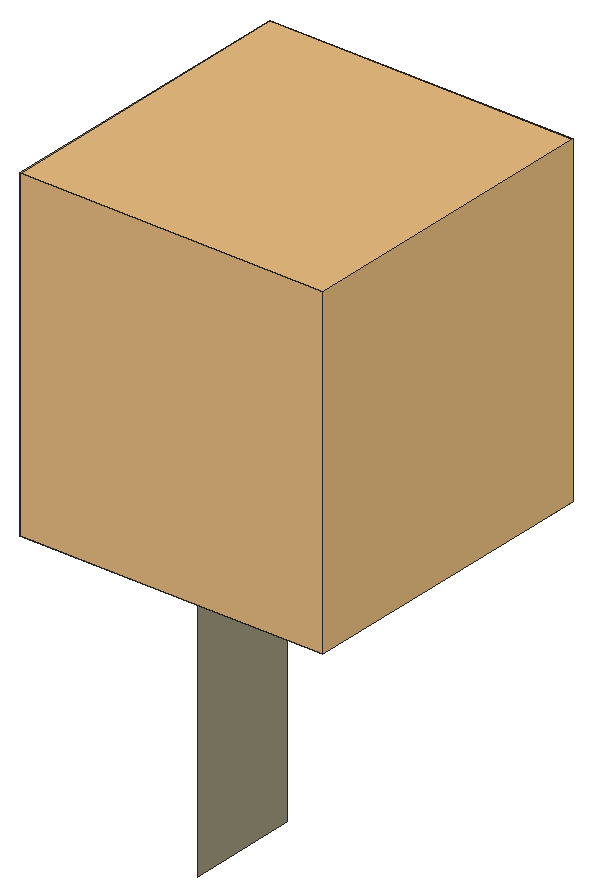
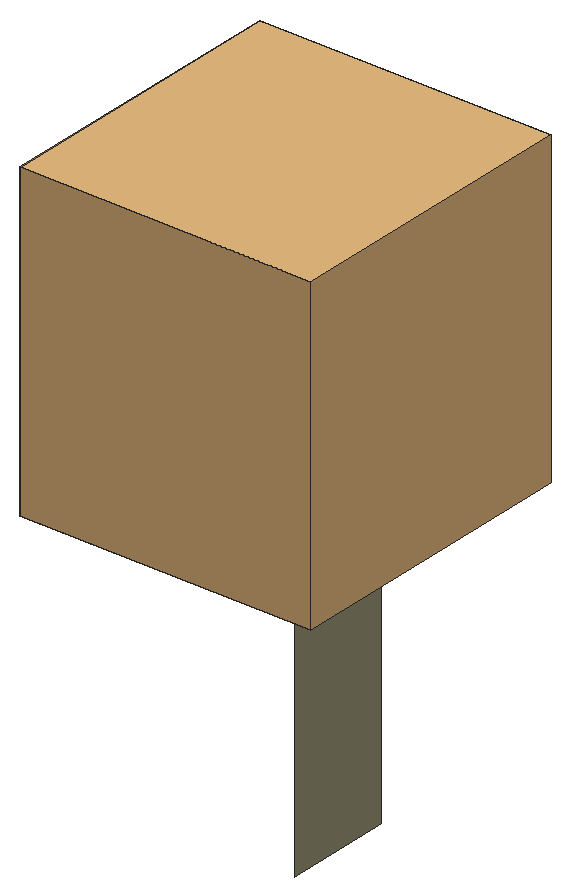
# SketchUp Ruby script. Lengths in inches.
U = 1.inch
M = Sketchup.active_model
def pt(a) = Geom::Point3d.new(a.map { |v| v * U })
def face(e, loops, mat)
  f = e.add_face(loops[0].map { |a| pt(a) })
  loops[1..].each { |l| e.add_face(l.map { |a| pt(a) }).erase! }
  f.material = f.back_material = mat if mat
  f
end
# faces: each face lists its corners as indices into pts; further lists are holes
def faces(e, pts, list, mat = nil) = list.each { |f| face(e, (f[0].is_a?(Array) ? f : [f]).map { |l| l.map { |i| pts[i] } }, mat) }
# xy, xz, yz: faces in a plane at the given z, y or x. An outline is a flat list of corners, or four numbers for a rectangle; further outlines are holes
def ring(l) = l.size == 4 ? [[l[0], l[1]], [l[2], l[1]], [l[2], l[3]], [l[0], l[3]]] : l.each_slice(2).to_a
def flat(e, list, mat, &to3) = list.each { |f| face(e, (f[0].is_a?(Array) ? f : [f]).map { |l| ring(l).map { |u, v| to3.(u, v) } }, mat) }
def xy(e, z, list, mat = nil) = flat(e, list, mat) { |x, y| [x, y, z] }
def xz(e, y, list, mat = nil) = flat(e, list, mat) { |x, z| [x, y, z] }
def yz(e, x, list, mat = nil) = flat(e, list, mat) { |y, z| [x, y, z] }
def lines(e, pts, list) = list.each { |a, b| e.add_line(pt(pts[a]), pt(pts[b])) }
# prism: a flat outline (further loops are holes) pulled along v
def prism(e, loops, v, mat = nil)
  f = face(e, loops, mat); d = Geom::Vector3d.new(v.map { |x| x * U })
  f.pushpull(f.normal.samedirection?(d) ? d.length : -d.length)
end
def box(e, o, s, mat = nil) = prism(e, [[o, [o[0] + s[0], o[1], o[2]], [o[0] + s[0], o[1] + s[1], o[2]], [o[0], o[1] + s[1], o[2]]]], [0, 0, s[2]], mat)
def at(x, y, z, deg = 0) = Geom::Transformation.translation(pt([x, y, z])) * Geom::Transformation.rotation(ORIGIN, Z_AXIS, deg.degrees)
def axes(o, x, y, z) = Geom::Transformation.new([*x, 0, *y, 0, *z, 0, *pt(o).to_a, 1])
def part(name) = M.definitions.add(name)
# library, detail: a bought-in or finely detailed component or shape, given as its bounding box
def library(name, o, s) = part(name).tap { |d| box(d.entities, o, s) }
def detail(e, o, s) = box(e.add_group.entities, o, s)
def put(e, d, t, mat = nil) = e.add_instance(d, t).tap { |i| i.material = mat if mat }
def group(e, t, mat = nil) = e.add_group.tap { |g| g.transformation = t; g.material = mat if mat }.entities
root = M.entities
M.materials.add("[Stone Coursed Rough]").color = [155, 150, 122]
c1 = library("chau cay",[-24.34,-109.24,0],[56.46,62.58,79.69])
yz(root,281.86,[[203.17,96.63,217.98,130.875]],"[Stone Coursed Rough]")
put(root,c1,axes([285.73,262.6875,137.875],[0.71,0,0],[0,0.66,0],[0,0,0.5396]))
